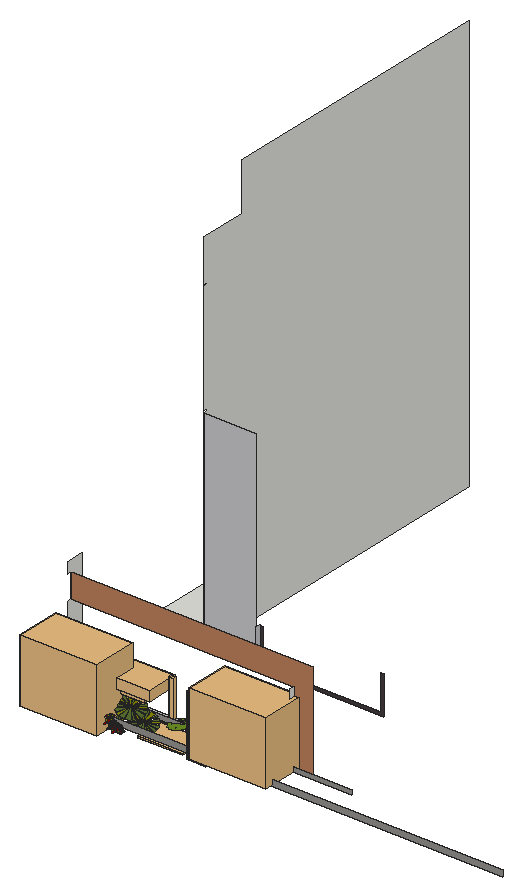
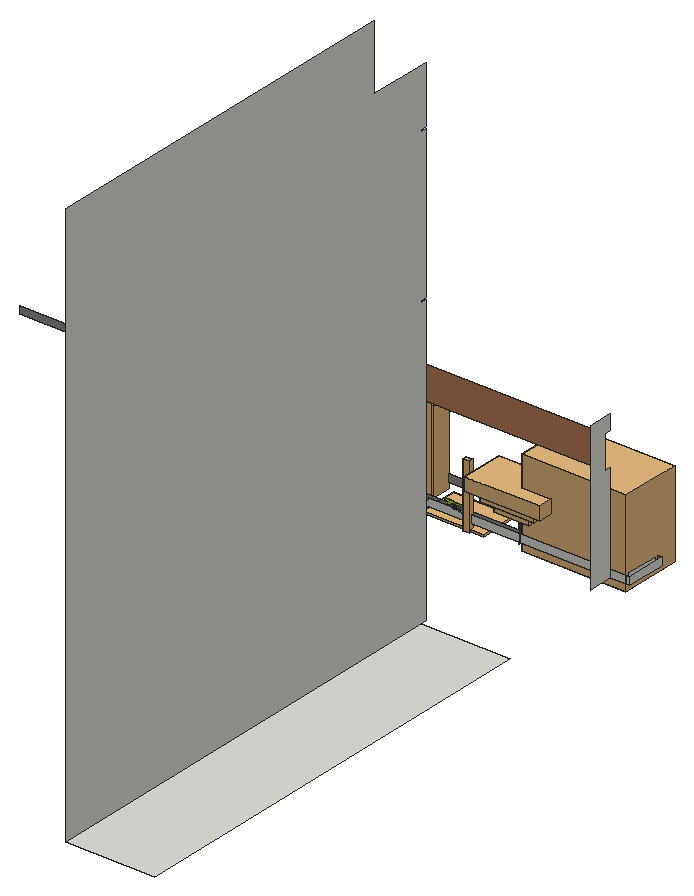
# SketchUp Ruby script. Lengths in inches.
U = 1.inch
M = Sketchup.active_model
def pt(a) = Geom::Point3d.new(a.map { |v| v * U })
def face(e, loops, mat)
  f = e.add_face(loops[0].map { |a| pt(a) })
  loops[1..].each { |l| e.add_face(l.map { |a| pt(a) }).erase! }
  f.material = f.back_material = mat if mat
  f
end
# faces: each face lists its corners as indices into pts; further lists are holes
def faces(e, pts, list, mat = nil) = list.each { |f| face(e, (f[0].is_a?(Array) ? f : [f]).map { |l| l.map { |i| pts[i] } }, mat) }
# xy, xz, yz: faces in a plane at the given z, y or x. An outline is a flat list of corners, or four numbers for a rectangle; further outlines are holes
def ring(l) = l.size == 4 ? [[l[0], l[1]], [l[2], l[1]], [l[2], l[3]], [l[0], l[3]]] : l.each_slice(2).to_a
def flat(e, list, mat, &to3) = list.each { |f| face(e, (f[0].is_a?(Array) ? f : [f]).map { |l| ring(l).map { |u, v| to3.(u, v) } }, mat) }
def xy(e, z, list, mat = nil) = flat(e, list, mat) { |x, y| [x, y, z] }
def xz(e, y, list, mat = nil) = flat(e, list, mat) { |x, z| [x, y, z] }
def yz(e, x, list, mat = nil) = flat(e, list, mat) { |y, z| [x, y, z] }
def lines(e, pts, list) = list.each { |a, b| e.add_line(pt(pts[a]), pt(pts[b])) }
# prism: a flat outline (further loops are holes) pulled along v
def prism(e, loops, v, mat = nil)
  f = face(e, loops, mat); d = Geom::Vector3d.new(v.map { |x| x * U })
  f.pushpull(f.normal.samedirection?(d) ? d.length : -d.length)
end
def box(e, o, s, mat = nil) = prism(e, [[o, [o[0] + s[0], o[1], o[2]], [o[0] + s[0], o[1] + s[1], o[2]], [o[0], o[1] + s[1], o[2]]]], [0, 0, s[2]], mat)
def at(x, y, z, deg = 0) = Geom::Transformation.translation(pt([x, y, z])) * Geom::Transformation.rotation(ORIGIN, Z_AXIS, deg.degrees)
def axes(o, x, y, z) = Geom::Transformation.new([*x, 0, *y, 0, *z, 0, *pt(o).to_a, 1])
def part(name) = M.definitions.add(name)
# library, detail: a bought-in or finely detailed component or shape, given as its bounding box
def library(name, o, s) = part(name).tap { |d| box(d.entities, o, s) }
def detail(e, o, s) = box(e.add_group.entities, o, s)
def put(e, d, t, mat = nil) = e.add_instance(d, t).tap { |i| i.material = mat if mat }
def group(e, t, mat = nil) = e.add_group.tap { |g| g.transformation = t; g.material = mat if mat }.entities
root = M.entities
M.materials.add("[0022_Maroon]").color = [128, 0, 0]
M.materials.add("[0043_SaddleBrown]").color = [139, 69, 19]
M.materials.add("[0058_Olive]").color = [128, 128, 0]
M.materials.add("[0059_DarkOliveGreen]").color = [85, 107, 47]
M.materials.add("[0061_OliveDrab]").color = [107, 142, 35]
M.materials.add("[Asphalt New]").color = [67, 60, 62]
M.materials.add("[Granite Light Gray]").color = [149, 148, 144]
M.materials.add("[Polished Concrete New]").color = [200, 200, 203]
M.materials.add("[Wood Veneer 02]").color = [190, 128, 91]
c1 = library("EXOTIC-KENTIA\#1",[0.7,-0.7,-0.11],[104.19,106.14,86.09])
c2 = part("Group\#46")
p = [[0.46,5.4,1.48],[0.55,4.86,1.35],[0.68,4.33,1.23],[0.85,3.8,1.12],[1.04,3.28,1.02],[1.28,2.78,0.93],
  [1.54,2.29,0.84],[1.84,1.82,0.77],[2.17,1.36,0.71],[2.52,0.93,0.66],[2.91,0.52,0.62],[2.91,0,0.48],
  [2.47,0.44,0.52],[2.06,0.9,0.56],[1.68,1.39,0.625],[1.34,1.9,0.7],[1.03,2.43,0.79],[0.76,2.98,0.89],
  [0.53,3.55,1],[0.34,4.13,1.12],[0.19,4.72,1.25],[0.09,5.3125,1.39],[0.02,5.91,1.54],[0,6.51,1.69],
  [0.02,6.88,1.8],[0.1,7.24,1.91],[0.22,7.59,2.02],[0.39,7.92,2.14],[0.6,8.22,2.26],[0.85,8.49,2.38],
  [1.14,8.72,2.49],[1.45,8.91,2.6],[1.8,9.0625,2.71],[2.16,9.17,2.8],[2.53,9.22,2.88],[2.91,9.23,2.95],
  [2.91,4.61,1.72],[2.68,3.89,1.48],[2.18,2.26,0.95],[2.59,5.625,1.93],[1.61,4.02,1.32],[2.34,6.73,2.18],
  [1.25,5.66,1.69],[2.4,7.87,2.5],[1.14,7.72,2.22],[2.4375,8.83,2.76],[2.16,8.77,2.69],[1.89,8.68,2.62],
  [1.625,8.56,2.54],[1.39,8.42,2.46],[1.16,8.24,2.37],[0.97,8.04,2.28],[0.79,7.82,2.19],[0.65,7.58,2.1],
  [0.54,7.32,2.01],[0.45,7.05,1.92],[0.4,6.78,1.84],[0.39,6.49,1.76],[0.41,5.95,1.62],[5.79,6.88,1.8],
  [5.82,6.51,1.69],[5.79,5.91,1.54],[5.73,5.3125,1.39],[5.625,4.72,1.25],[5.48,4.13,1.12],[5.29,3.55,1],
  [5.06,2.98,0.89],[4.79,2.43,0.79],[4.48,1.9,0.7],[4.14,1.39,0.625],[3.76,0.9,0.56],[3.35,0.44,0.52],
  [3.29,0.93,0.66],[3.65,1.36,0.71],[3.98,1.82,0.77],[4.27,2.29,0.84],[4.54,2.78,0.93],[4.77,3.28,1.02],
  [4.97,3.8,1.12],[5.13,4.33,1.23],[5.26,4.86,1.35],[5.35,5.4,1.48],[5.41,5.95,1.62],[5.43,6.49,1.76],
  [5.41,6.78,1.84],[5.36,7.05,1.92],[5.28,7.32,2.01],[5.16,7.58,2.1],[5.02,7.82,2.19],[4.85,8.04,2.28],
  [4.65,8.24,2.37],[4.43,8.42,2.46],[4.1875,8.56,2.54],[3.93,8.68,2.62],[3.66,8.77,2.69],[3.38,8.83,2.76],
  [4.67,7.72,2.22],[3.41,7.87,2.5],[4.5625,5.66,1.69],[3.47,6.73,2.18],[4.21,4.02,1.32],[3.23,5.625,1.93],
  [3.64,2.26,0.95],[3.13,3.89,1.48],[3.29,9.22,2.88],[3.66,9.17,2.8],[4.02,9.0625,2.71],[4.36,8.91,2.6],
  [4.68,8.72,2.49],[4.96,8.49,2.38],[5.21,8.22,2.26],[5.43,7.92,2.14],[5.59,7.59,2.02],[5.72,7.24,1.91],
  [2.91,14.34,0]]
faces(c2.entities,p,[[0,1,2,3,4,5,6,7,8,9,10,11,12,13,14,15,16,17,18,19,20,21,22,23,24,25,26,27,28,29,30,31,32,33,34,35,36,10,37,38,39,40,41,42,43,44,45,46,47,48,49,50,51,52,53,54,55,56,57,58],[59,60,61,62,63,64,65,66,67,68,69,70,71,11,10,72,73,74,75,76,77,78,79,80,81,82,83,84,85,86,87,88,89,90,91,92,93,94,95,96,97,98,99,100,101,102,103,10,36,35,104,105,106,107,108,109,110,111,112,113]],"[0022_Maroon]")
faces(c2.entities,p,[[43,42,41,40,39,38,37,10,9,8,7,6,5,4,3,2,1,0,58,57,56,55,54,53,52,51,50,49,48,47,46,45,44],[99,98,97,96,95,94,93,92,91,90,89,88,87,86,85,84,83,82,81,80,79,78,77,76,75,74,73,72,10,103,102,101,100]],"[0058_Olive]")
lines(c2.entities,p,[[35,114]])
c3 = part("EXOTIC-CROTON")
p = [[0,0,13.11],[0,0,0],[0,0,17.6]]
lines(c3.entities,p,[[0,1],[0,2]])
put(c3.entities,c2,at(-2.91,-14.34,9.43),"[0058_Olive]")
put(c3.entities,c2,at(-13.875,-4.65,9.43,-60),"[0058_Olive]")
put(c3.entities,c2,at(-10.97,9.69,9.43,-120),"[0058_Olive]")
put(c3.entities,c2,at(2.91,14.34,9.43,180),"[0058_Olive]")
put(c3.entities,c2,at(13.875,4.65,9.43,120),"[0058_Olive]")
put(c3.entities,c2,at(10.97,-9.69,9.43,60),"[0058_Olive]")
put(c3.entities,c2,axes([-3.96,11.79,13.11],[-0.73612,-0.425,0],[0.425,-0.73612,0],[0,0,0.85]),"[0058_Olive]")
put(c3.entities,c2,axes([8.24,9.32,13.11],[-0.73612,0.425,0],[-0.425,-0.73612,0],[0,0,0.85]),"[0058_Olive]")
put(c3.entities,c2,axes([3.96,-11.79,13.11],[0.73612,0.425,0],[-0.425,0.73612,0],[0,0,0.85]),"[0058_Olive]")
put(c3.entities,c2,axes([-8.24,-9.32,13.11],[0.73612,-0.425,0],[0.425,0.73612,0],[0,0,0.85]),"[0058_Olive]")
put(c3.entities,c2,axes([12.19,-2.47,13.11],[0,0.85,0],[-0.85,0,0],[0,0,0.85]),"[0058_Olive]")
put(c3.entities,c2,axes([-12.19,2.47,13.11],[0,-0.85,0],[0.85,0,0],[0,0,0.85]),"[0058_Olive]")
put(c3.entities,c2,axes([1.98,9.75,17.6],[-0.68,0,0],[0,-0.68,0],[0,0,0.68]),"[0058_Olive]")
put(c3.entities,c2,axes([7.46,-6.59,17.6],[0.34,0.5889,0],[-0.5889,0.34,0],[0,0,0.68]),"[0058_Olive]")
put(c3.entities,c2,axes([9.4375,3.16,17.6],[-0.34,0.5889,0],[-0.5889,-0.34,0],[0,0,0.68]),"[0058_Olive]")
put(c3.entities,c2,axes([-9.4375,-3.16,17.6],[0.34,-0.5889,0],[0.5889,0.34,0],[0,0,0.68]),"[0058_Olive]")
put(c3.entities,c2,axes([-7.46,6.59,17.6],[-0.34,-0.5889,0],[0.5889,-0.34,0],[0,0,0.68]),"[0058_Olive]")
put(c3.entities,c2,axes([-1.98,-9.75,17.6],[0.68,0,0],[0,0.68,0],[0,0,0.68]),"[0058_Olive]")
c4 = part("Group\#44")
p = [[12.14,1.93,0.52],[12.15,1.96,0.53]]
lines(c4.entities,p,[[0,1]])
detail(c4.entities,[0,0,0],[22.29,22.29,3.9])
c5 = part("EXOTIC-BUSHY-02")
prism(c5.entities,[[[-0.2,0.11,-0.03],[-0.16,0.16,-0.03],[-0.11,0.2,-0.03],[-0.06,0.22,-0.03],[0,0.23,-0.03],[0.06,0.22,-0.03],[0.11,0.2,-0.03],[0.16,0.16,-0.03],[0.2,0.11,-0.03],[0.22,0.06,-0.03],[0.23,0,-0.03],[0.22,-0.06,-0.03],[0.2,-0.11,-0.03],[0.16,-0.16,-0.03],[0.11,-0.2,-0.03],[0.06,-0.22,-0.03],[0,-0.23,-0.03],[-0.06,-0.22,-0.03],[-0.11,-0.2,-0.03],[-0.16,-0.16,-0.03],[-0.2,-0.11,-0.03],[-0.22,-0.06,-0.03],[-0.23,0,-0.03],[-0.22,0.06,-0.03]]],[0,0,12.79],"[0043_SaddleBrown]")
put(c5.entities,c4,axes([-11.15,-11.15,16.66],[1,0,0],[0,1,0],[0,0,-1]))
put(c5.entities,c4,axes([-7.91,-7.91,13.14],[0.71,0,0],[0,0.71,0],[0,0,-0.71]))
put(c5.entities,c4,axes([-5.11,-5.11,9.7],[0.4588,0,0],[0,0.4588,0],[0,0,-0.4588]))
c6 = part("Group\#77")
p = [[9.84,8.91,4.16],[6.8,0.43,0.2],[7.02,0.37,0.17],[7.24,0.3125,0.15],[7.46,0.26,0.12],[7.68,0.21,0.1],
  [7.91,0.17,0.08],[8.13,0.13,0.0625],[8.36,0.1,0.04],[8.59,0.07,0.03],[8.8125,0.04,0.02],[9.04,0.02,0.01],
  [9.27,0.01,0],[9.5,0,0],[10.87,0.04,0.02],[11.1,0.07,0.03],[11.33,0.1,0.04],[11.55,0.13,0.0625],
  [11.78,0.17,0.08],[12,0.21,0.1],[12.22,0.26,0.12],[12.45,0.3125,0.15],[12.67,0.37,0.17],[12.88,0.43,0.2],
  [13.1,0.5,0.23],[13.32,0.57,0.27],[13.53,0.64,0.3],[4.34,1.52,0.71],[4.43,1.46,0.68],[4.53,1.41,0.66],
  [4.625,1.35,0.63],[4.72,1.3,0.6],[4.82,1.24,0.58],[4.92,1.19,0.55],[5.02,1.14,0.53],[5.12,1.09,0.51],
  [5.22,1.04,0.48],[5.32,0.99,0.46],[5.43,0.94,0.44],[5.53,0.9,0.42],[14.76,1.19,0.55],[14.86,1.24,0.58],
  [14.96,1.3,0.6],[15.06,1.35,0.63],[15.16,1.41,0.66],[15.25,1.46,0.68],[15.35,1.52,0.71],[15.44,1.58,0.74],
  [15.53,1.64,0.76],[15.63,1.7,0.79],[15.72,1.76,0.82],[15.8125,1.82,0.85],[15.9,1.89,0.88],[1.5,4.1875,1.95],
  [1.62,4.01,1.87],[1.75,3.84,1.79],[1.88,3.67,1.71],[2.02,3.51,1.63],[2.16,3.34,1.56],[2.3,3.18,1.48],
  [2.45,3.02,1.41],[2.61,2.87,1.34],[2.76,2.72,1.27],[2.92,2.57,1.2],[3.09,2.43,1.13],[3.26,2.29,1.07],
  [17.81,3.67,1.71],[17.74,3.59,1.67],[17.67,3.51,1.63],[17.6,3.42,1.6],[17.53,3.34,1.56],[17.46,3.26,1.52],
  [17.38,3.18,1.48],[17.31,3.1,1.45],[17.23,3.02,1.41],[17.16,2.95,1.375],[17.08,2.87,1.34],[17,2.79,1.3],
  [16.92,2.72,1.27],[18.53,4.73,2.2],[18.64,4.91,2.29],[18.74,5.1,2.38],[18.83,5.29,2.47],[18.92,5.48,2.55],
  [19.01,5.67,2.64],[19.09,5.86,2.73],[19.17,6.06,2.83],[19.24,6.26,2.92],[19.3,6.46,3.01],[19.36,6.66,3.1],
  [19.42,6.86,3.2],[19.47,7.06,3.29],[0.1,7.67,3.58],[0.13,7.47,3.48],[0.17,7.26,3.39],[0.22,7.06,3.29],
  [0.27,6.86,3.2],[0.32,6.66,3.1],[0.38,6.46,3.01],[0.45,6.26,2.92],[0.52,6.06,2.83],[0.59,5.86,2.73],
  [0.67,5.67,2.64],[0.76,5.48,2.55],[0.85,5.29,2.47],[19.66,8.29,3.87],[19.67,8.5,3.96],[19.68,8.71,4.06],
  [19.69,8.91,4.16],[19.68,9.12,4.25],[19.67,9.33,4.35],[19.66,9.54,4.45],[19.64,9.74,4.54],[19.62,9.95,4.64],
  [19.59,10.16,4.74],[19.55,10.36,4.83],[19.51,10.57,4.93],[19.47,10.77,5.02],[0.1,10.16,4.74],[0.08,10.05,4.6875],
  [0.07,9.95,4.64],[0.05,9.85,4.59],[0.04,9.74,4.54],[0.03,9.64,4.5],[0.02,9.54,4.45],[0.02,9.43,4.4],
  [0.01,9.33,4.35],[0.01,9.23,4.3],[0,9.12,4.25],[0,9.02,4.21],[0,8.91,4.16],[0.85,12.54,5.85],
  [0.8,12.45,5.8],[0.76,12.35,5.76],[0.72,12.26,5.72],[0.67,12.16,5.67],[0.63,12.0625,5.625],[0.59,11.97,5.58],
  [0.56,11.87,5.53],[0.52,11.77,5.49],[0.48,11.67,5.44],[0.45,11.57,5.4],[0.41,11.47,5.35],[0.38,11.375,5.3],
  [3.26,15.54,7.25],[3.09,15.4,7.18],[2.92,15.26,7.12],[2.76,15.11,7.05],[2.61,14.96,6.98],[2.45,14.81,6.9],
  [2.3,14.65,6.83],[2.16,14.49,6.76],[2.02,14.32,6.68],[1.88,14.16,6.6],[1.75,13.99,6.52],[1.62,13.82,6.44],
  [1.5,13.64,6.36],[6.8,17.4,8.11],[6.58,17.33,8.08],[6.37,17.26,8.05],[6.16,17.1875,8.01],[5.94,17.11,7.98],
  [5.73,17.02,7.9375],[5.53,16.93,7.9],[5.32,16.84,7.85],[5.12,16.74,7.81],[4.92,16.64,7.76],[4.72,16.53,7.71],
  [4.53,16.42,7.66],[4.34,16.31,7.61],[9.5,17.83,8.3125],[9.38,17.83,8.3125],[9.27,17.82,8.31],[9.16,17.8125,8.31],
  [9.04,17.81,8.3],[8.93,17.8,8.3],[8.8125,17.79,8.29],[8.7,17.77,8.29],[8.59,17.76,8.28],[8.47,17.75,8.28],
  [8.36,17.73,8.27],[8.25,17.72,8.26],[8.13,17.7,8.25],[19.09,11.97,5.58],[19.05,12.0625,5.625],[19.01,12.16,5.67],
  [18.97,12.26,5.72],[18.92,12.35,5.76],[18.88,12.45,5.8],[18.83,12.54,5.85],[18.79,12.64,5.89],[18.74,12.73,5.9375],
  [18.6875,12.83,5.98],[18.64,12.92,6.02],[18.59,13.01,6.07],[18.53,13.1,6.11],[16.92,15.11,7.05],[17,15.04,7.01],
  [17.08,14.96,6.98],[17.16,14.88,6.94],[17.23,14.81,6.9],[17.31,14.73,6.87],[17.38,14.65,6.83],[17.46,14.57,6.79],
  [17.53,14.49,6.76],[17.6,14.41,6.72],[17.67,14.32,6.68],[17.74,14.24,6.64],[17.81,14.16,6.6],[15.9,15.94,7.43],
  [15.8125,16.01,7.46],[15.72,16.07,7.49],[15.63,16.13,7.52],[15.53,16.19,7.55],[15.44,16.25,7.58],[15.35,16.31,7.61],
  [15.25,16.37,7.63],[15.16,16.42,7.66],[15.06,16.48,7.68],[14.96,16.53,7.71],[14.86,16.59,7.73],[14.76,16.64,7.76],
  [13.53,17.1875,8.01],[13.32,17.26,8.05],[13.1,17.33,8.08],[12.88,17.4,8.11],[12.67,17.46,8.14],[12.45,17.52,8.17],
  [12.22,17.57,8.19],[12,17.62,8.22],[11.78,17.66,8.24],[11.55,17.7,8.25],[11.33,17.73,8.27],[11.1,17.76,8.28],
  [10.87,17.79,8.29]]
faces(c6.entities,p,[[0,1,2,3,4,5,6,7,8,9,10,11,12,13],[0,14,15,16,17,18,19,20,21,22,23,24,25,26],[0,40,41,42,43,44,45,46,47,48,49,50,51,52],[0,53,54,55,56,57,58,59,60,61,62,63,64,65],[0,79,80,81,82,83,84,85,86,87,88,89,90,91],[0,92,93,94,95,96,97,98,99,100,101,102,103,104],[0,105,106,107,108,109,110,111,112,113,114,115,116,117],[0,118,119,120,121,122,123,124,125,126,127,128,129,130],
  [0,144,145,146,147,148,149,150,151,152,153,154,155,156],[0,170,171,172,173,174,175,176,177,178,179,180,181,182],[0,196,197,198,199,200,201,202,203,204,205,206,207,208],[0,209,210,211,212,213,214,215,216,217,218,219,220,221]],"[0059_DarkOliveGreen]")
faces(c6.entities,p,[[0,27,28,29,30,31,32,33,34,35,36,37,38,39],[0,66,67,68,69,70,71,72,73,74,75,76,77,78],[0,131,132,133,134,135,136,137,138,139,140,141,142,143],[0,157,158,159,160,161,162,163,164,165,166,167,168,169],[0,183,184,185,186,187,188,189,190,191,192,193,194,195],[0,222,223,224,225,226,227,228,229,230,231,232,233,234]],"[0058_Olive]")
c7 = part("EXOTIC-AUS-PALM")
put(c7.entities,c6,axes([-13.78,-12.48,-5.82],[1.4,0,0],[0,1.4,0],[0,0,1.4]))
put(c7.entities,c6,at(-21.65,-8.91,-12.03))
put(c7.entities,c6,axes([-1.28,-11.86,-13.4],[1.33,0,0],[0,1.33,0],[0,0,1.33]))
c8 = library("EXOTIC-BULLRUSH",[-0.59,-0.59,-0.94],[7.09,7.09,64.29])
c9 = library("EXOTIC-AMAZON-LILY",[-1.1,-0.12,0],[60.56,66.69,1.97])
c10 = library("EXOTICA-CAT-TAIL",[-18.64,-20.64,0],[26.41,31.25,82.25])
c11 = library("EXOTIC-BAMBOO-TOO",[-9.25,-15.15,0],[30.31,37.46,85.46])
c12 = library("EXOTIC-BAMBOO",[-8.14,-8.14,0],[38.48,34.74,73.65])
c13 = library("EXOTIC-PEONY",[-0.63,-0.48,-0.08],[13.23,10.24,55.71])
c14 = library("EXOTIC-RED-POKER\#1",[-1.18,-1.18,0],[10.24,10.24,66.04])
xy(root,0,[[0,304.24,88.9375,747.375]])
xz(root,114.25,[[0,0,641.18,7.8125]],"[Granite Light Gray]")
xz(root,150.16,[[3.82,0.6875,408.3,7.8125]],"[Granite Light Gray]")
xz(root,153.99,[[0,0,20.0625,7.8125],[20.0625,0,321.78,7.8125]])
xz(root,160.36,[[321.78,0,347.76,0,347.76,131.1875,20.0625,131.1875,20.0625,97.93,321.78,97.93]],"[Wood Veneer 02]")
xz(root,298.43,[[88.9375,0,160.07,287.46]],"[Polished Concrete New]")
xz(root,304.24,[[160.07,0,328.15,0,328.15,52.25,323.93,52.25,323.93,4.22,164.29,4.22,164.29,52.25,160.07,52.25]],"[Asphalt New]")
yz(root,0,[[114.25,0,153.99,7.8125]])
yz(root,3.82,[[118.08,0.6875,150.16,7.8125]])
yz(root,20.0625,[[153.99,0,153.99,97.93,160.36,97.93,160.36,131.1875,153.99,131.1875,153.99,146.4375,178.37,146.4375,178.37,0]])
yz(root,88.9375,[[298.43,0,298.43,287.46,304.24,287.46,304.24,289.58,298.43,289.58,298.43,440.86,304.24,440.86,304.24,442.55,298.43,442.55,298.43,500.25,363.07,500.25,363.07,566.3125,747.375,566.3125,747.375,0]])
yz(root,160.07,[[298.43,0,304.24,52.25]],"[Polished Concrete New]")
yz(root,321.78,[[153.99,0,160.36,97.93]])
p = [[193.92,154,8.05],[192.73,153.86,8.3],[192.01,151.875,7.59],[192.05,150.6875,7.05],[192.66,150,6.58],[193.37,149.66,6.25],
  [192.67,148.58,5.94],[193.09,147.58,5.39],[193.85,147.02,4.9375],[195.28,146.53,4.35],[195.76,146.3,4.125],[195.85,147.5,4.64],
  [196.51,148.72,5.02],[197.52,149.89,5.28],[198.78,150.74,5.34],[199.17,150.9,5.3125],[199.31,150.84,5.25],[199.15,150.55,5.16],
  [197.87,149.16,4.87],[197.03,147.93,4.53],[196.34,146.61,4.12],[196.13,145.91,3.85],[196.44,145.3,3.5],[197.15,144.97,3.17],
  [198.34,144.62,2.71],[199.42,144.32,2.29],[199.98,144.17,2.08],[200.91,143.625,1.6],[201.99,143.24,1.15],[203.08,143.01,0.76],
  [203.66,142.85,0.54],[203.58,143.52,0.86],[203.47,144.52,1.34],[204.58,142.73,0.25],[204.89,142.51,0.08],[205.9,142.45,-0.21],
  [206.92,142.39,-0.5],[209.25,142.85,-0.89],[212.55,143.08,-1.64],[213.89,144.1875,-1.49],[215.22,144.97,-1.48],[216.08,145.4,-1.51],
  [214.42,146.54,-0.57],[213.12,147.16,0.04],[211.25,147.59,0.72],[209.94,147.85,1.17],[209.29,148.16,1.48],[208.77,148.41,1.72],
  [208.77,148.58,1.8],[209.125,148.63,1.73],[210.16,148.5,1.41],[211.04,148.28,1.08],[212.85,147.59,0.31],[214.37,146.96,-0.37],
  [215.33,146.62,-0.77],[215.96,146.21,-1.11],[216.43,145.78,-1.43],[217.11,146.45,-1.3],[217.43,147.02,-1.13],[217.6,147.54,-0.94],
  [217.68,147.94,-0.78],[217.85,148.42,-0.61],[216.36,149.31,0.17],[214.95,149.78,0.75],[213.71,150,1.16],[211.41,150.24,1.87],
  [209.65,150.3125,2.35],[208.16,150.42,2.78],[207.05,150.5625,3.13],[206.52,150.81,3.38],[206.49,151.15,3.54],[207.32,151.3,3.39],
  [208.46,151.39,3.14],[210.46,151.22,2.55],[212.61,150.79,1.8],[214.99,150.12,0.89],[217.67,149.09,-0.26],[217.97,150.81,0.43],
  [218.01,151.83,0.88],[217.59,152.27,1.1875],[216.61,152.74,1.65],[215.4,153.01,2.08],[213.78,153.12,2.55],[212.4,153.19,2.93],
  [210.36,153.28,3.5],[208.85,153.22,3.86],[207.67,153.17,4.14],[207.1,153.11,4.26],[206.77,153.26,4.42],[207.12,153.5,4.43],
  [207.99,153.81,4.34],[209.36,153.95,4.06],[212.13,153.83,3.29],[213.76,153.64,2.78],[215.21,153.38,2.3],[215.88,153.14,2.01],
  [217.22,152.74,1.49],[217.27,153.03,1.61],[216.9375,154.02,2.14],[216.59,154.9,2.625],[215.24,155.9,3.42],[213.83,156.09,3.87],
  [211.57,155.95,4.39],[209.58,155.53,4.71],[207.77,155.23,5.04],[206.97,155.07,5.18],[206.52,155.1,5.3],[206.57,155.28,5.37],
  [207.49,155.65,5.3],[209.72,156.18,4.96],[211.52,156.33,4.57],[214.4,156.32,3.83],[212.95,157.51,4.73],[211.49,158.13,5.39],
  [210.26,158.24,5.75],[209.625,158.04,5.82],[207.72,157.38,6.02],[206.31,156.77,6.11],[205.2,156.39,6.22],[204.75,156.35,6.32],
  [204.61,156.51,6.43],[204.85,156.68,6.44],[206.63,157.48,6.34],[208.06,157.93,6.18],[209.33,158.23,5.98],[210.3,158.43,5.83],
  [209.11,158.87,6.33],[208,159,6.67],[206.57,158.8125,6.96],[205.23,158.43,7.13],[203.86,158.16,7.36],[203.15,157.68,7.33],
  [201.97,157.09,7.37],[200.96,156.41,7.32],[200.48,155.5,7.04],[200.62,154.56,6.58],[200.96,154.01,6.25],[200.28,153.81,6.33],
  [199.7,154.26,6.68],[198.73,154.72,7.14],[197.46,154.69,7.45],[195.61,154.35,7.77],[197.42,152.83,6.63],[193.95,152.56,7.4],
  [196.18,152.94,7],[200.84,153.75,6.16],[201.41,154.45,6.33],[202.3125,155.95,6.77],[203.5,156.88,6.88],[204.52,157.43,6.86],
  [202.93,155.86,6.57],[202,154.56,6.22],[201.71,153.83,5.97],[203.01,154.99,6.16],[205.59,156.09,5.99],[207.64,156.66,5.72],
  [209.76,157.11,5.375],[210.83,157.25,5.16],[207.55,156.34,5.6],[205.6,155.7,5.8125],[203.45,154.83,5.97],[202.34,154.08,5.92],
  [201.88,153.66,5.85],[201.99,153.39,5.7],[202.34,153.34,5.59],[203.29,153.59,5.46],[204.25,154,5.39],[205.375,154.27,5.23],
  [208.64,154.79,4.62],[210.73,154.95,4.16],[212.68,154.8,3.59],[214.27,154.7,3.13],[214.86,154.42,2.85],[211.81,154.625,3.73],
  [210.08,154.56,4.15],[207.35,154.27,4.72],[204.94,153.77,5.11],[202.31,153.1,5.49],[203.68,152.03,4.66],[205.72,152.29,4.25],
  [207.64,152.49,3.85],[211.61,152.29,2.73],[213.58,151.92,2.06],[214.9,151.59,1.57],[215.52,151.3,1.28],[213.65,151.65,1.92],
  [210.58,151.96,2.85],[206.65,152.0625,3.91],[204.3,151.74,4.37],[206.4,149.69,2.91],[207.98,149.84,2.57],[209.92,149.64,1.98],
  [211.78,149.18,1.3],[213.18,148.7,0.72],[214.72,147.97,-0.01],[211.53,149,1.28],[209.69,149.42,1.94],[207.98,149.56,2.44],
  [206.42,149.45,2.8],[207.76,147.86,1.74],[209.47,147.57,1.17],[210.99,147.08,0.55],[212.24,146.48,-0.03],[212.79,145.9,-0.4375],
  [210.7,146.9,0.55],[209.13,147.3,1.13],[207.87,147.53,1.56],[209.17,146.29,0.67],[209.84,145.63,0.2],[210.82,144.78,-0.43],
  [210.64,144.89,-0.34],[208.76,146.14,0.7],[207.27,147.4,1.66],[206.14,148.92,2.63],[205.37,145.34,1.22],[205.38,149.42,3.05],
  [204.04,150.63,3.9375],[202.82,148.88,3.46],[201.58,146.05,2.51],[202.03,148.13,3.33],[202.94,150.0625,3.96],[203.68,151.08,4.23],
  [202.37,152.09,5.02],[200.23,149.89,4.58],[198.125,146.68,3.6875],[198.99,149.25,4.62],[200.47,150.95,5],[202.1,152.4,5.23],
  [201.66,152.82,5.53],[200.02,152.24,5.69],[197.84,151.48,5.91],[195.65,149.74,5.7],[197.15,151.3,6.01],[198.87,152.47,6.09],
  [200.81,152.92,5.8],[201.12,153.13,5.81],[200.48,153.43,6.11],[200.23,148.31,3.875],[200.96,149.49,4.22],[201.34,149.78,4.25],
  [201.61,149.85,4.21],[201.72,149.71,4.12],[201.5,149.24,3.97],[200.97,148.11,3.6],[200.4,146.87,3.1875],[199.96,145.5625,2.71],
  [199.73,144.95,2.5],[199.8,146.81,3.3125],[203.62,148.45,3.07],[203.97,148.875,3.17],[204.36,148.9,3.08],[204.58,148.71,2.9375],
  [204.61,148.3,2.74],[204.47,147.97,2.63],[203.96,146.66,2.17],[203.47,145.44,1.75],[203.4,147.3,2.61],[195.03,151.42,6.61],
  [196.01,151.94,6.59],[196.86,152.24,6.5],[197.32,152.21,6.375],[197.47,152.07,6.27],[196.04,151.18,6.24],[194.77,150.48,6.26],
  [194.4,150.35,6.29],[194.43,150.85,6.51],[204.02,153.2,5.09],[204.76,153.24,4.92],[205.3125,153.08,4.71],[205.26,152.86,4.625],
  [204.56,152.625,4.7],[203.7,152.68,4.94],[203.43,152.9375,5.13],[202.75,154.07,5.81],[203.51,154.26,5.7],[204.07,154.26,5.56],
  [204.05,154.04,5.46],[203.23,153.84,5.59],[202.625,153.82,5.73],[173.59,155.55,8.2],[171.69,155.95,7.89],[169.96,155.71,7.34],
  [168.98,155.28,6.89],[168.12,154.45,6.3],[167.73,154.18,6.08],[169.8125,154.125,6.59],[171.94,153.75,6.97],[173.99,153.17,7.23],
  [175.47,152.45,7.29],[175.75,152.22,7.26],[175.64,152.14,7.2],[175.13,152.23,7.11],[172.71,152.97,6.8125],[170.57,153.45,6.48],
  [168.27,153.85,6.07],[167.04,153.97,5.8],[165.99,153.79,5.45],[165.41,153.38,5.12],[164.79,152.7,4.66],[164.28,152.08,4.24],
  [164.02,151.76,4.03],[163.0625,151.22,3.55],[162.39,150.61,3.1],[161.98,149.98,2.71],[161.72,149.65,2.49],[162.875,149.7,2.8125],
  [164.63,149.76,3.29],[161.5,149.12,2.2],[161.125,148.94,2.03],[161.02,148.36,1.74],[160.91,147.78,1.45],[161.71,146.44,1.05],
  [162.11,144.55,0.3],[164.04,143.78,0.46],[165.4,143.02,0.47],[166.16,142.52,0.44],[168.14,143.48,1.38],[169.22,144.22,1.99],
  [169.97,145.29,2.66],[170.4375,146.05,3.12],[170.97,146.42,3.42],[171.4,146.72,3.67],[171.7,146.71,3.75],[171.79,146.51,3.68],
  [171.57,145.92,3.36],[171.18,145.42,3.03],[169.98,144.375,2.25],[168.88,143.51,1.58],[168.28,142.96,1.18],[167.57,142.59,0.83],
  [166.82,142.33,0.52],[167.99,141.93,0.65],[168.99,141.75,0.82],[169.88,141.65,1.01],[170.59,141.61,1.17],[171.43,141.51,1.34],
  [172.97,142.36,2.12],[173.79,143.17,2.7],[174.17,143.88,3.11],[174.6,145.21,3.82],[174.72,146.21,4.3],[174.91,147.07,4.73],
  [175.16,147.7,5.08],[175.6,148.01,5.33],[176.1875,148.02,5.49],[176.44,147.55,5.34],[176.6,146.89,5.09],[176.3,145.75,4.5],
  [175.56,144.51,3.75],[174.38,143.15,2.84],[172.58,141.61,1.68],[175.58,141.44,2.38],[177.36,141.42,2.83],[178.14,141.66,3.14],
  [178.96,142.22,3.6],[179.43,142.91,4.03],[179.61,143.84,4.49],[179.74,144.63,4.88],[179.9,145.8,5.45],[179.8,146.67,5.81],
  [179.71,147.35,6.09],[179.59,147.68,6.21],[179.87,147.87,6.37],[180.29,147.66,6.38],[180.8125,147.16,6.29],[181.07,146.375,6.01],
  [180.85,144.79,5.24],[180.52,143.86,4.73],[180.07,143.02,4.24],[179.65,142.64,3.96],[178.96,141.875,3.44],[179.46,141.84,3.56],
  [181.18,142.03,4.09],[182.72,142.23,4.57],[184.47,143.01,5.37],[184.8,143.82,5.82],[184.55,145.11,6.34],[183.82,146.25,6.66],
  [183.29,147.29,6.99],[183.02,147.75,7.125],[183.07,148.01,7.25],[183.38,147.98,7.32],[184.04,147.45,7.25],[184.95,146.17,6.91],
  [185.21,145.14,6.52],[185.2,143.49,5.77],[187.27,144.32,6.68],[188.36,145.16,7.34],[188.54,145.86,7.7],[188.19,146.23,7.77],
  [187.04,147.32,7.97],[185.99,148.13,8.06],[185.32,148.77,8.17],[185.24,149.02,8.27],[185.53,149.1,8.38],[185.82,148.96,8.39],
  [187.21,147.95,8.29],[188.01,147.125,8.13],[188.53,146.39,7.93],[188.88,145.84,7.78],[189.64,146.52,8.28],[189.87,147.16,8.62],
  [189.55,147.98,8.91],[188.87,148.75,9.08],[188.41,149.53,9.31],[187.57,149.94,9.28],[186.54,150.62,9.32],[185.35,151.2,9.27],
  [183.77,151.47,8.99],[182.13,151.39,8.53],[181.17,151.19,8.2],[180.82,151.59,8.28],[181.61,151.92,8.63],[182.42,152.48,9.09],
  [182.36,153.2,9.4],[181.76,154.26,9.72],[181.16,155.23,10],[180.9,155.92,10.24],[177.45,156.33,9.54],[175.38,156.31,9],
  [174.17,155.96,8.53],[168.39,152.82,5.63],[172.87,152.33,6.57],[175.84,151.48,6.95],[178.37,150.54,7.18],[179.1,150.79,7.48],
  [178.09,151.73,7.64],[176.76,152.98,7.86],[173.73,154.24,7.65],[176.45,153.38,7.96],[178.48,152.4,8.04],[179.27,151.28,7.74],
  [179.64,151.1,7.76],[180.16,151.47,8.06],[179.11,153.23,8.58],[178.64,155.22,9.35],[180.71,151.26,8.11],[181.93,150.9375,8.27],
  [184.54,150.42,8.71],[186.18,149.74,8.83],[187.125,149.15,8.8125],[184.39,150.07,8.52],[182.125,150.6,8.17],[180.86,150.77,7.92],
  [182.88,150.02,8.11],[184.79,148.54,7.9375],[185.8,147.36,7.67],[186.58,146.15,7.32],[186.82,145.54,7.11],[185.24,147.42,7.55],
  [184.12,148.54,7.76],[182.61,149.77,7.92],[181.29,150.41,7.87],[180.55,150.67,7.8],[180.09,150.61,7.65],[179.99,150.4,7.54],
  [180.44,149.86,7.41],[181.15,149.3125,7.34],[181.62,148.66,7.17],[182.53,146.79,6.57],[182.82,145.59,6.11],[182.55,144.47,5.53],
  [182.38,143.57,5.08],[181.88,143.22,4.8],[182.24,144.97,5.68],[182.13,145.96,6.09],[181.61,147.53,6.66],[180.76,148.91,7.0625],
  [179.58,150.42,7.4375],[177.72,149.64,6.61],[178.16,148.47,6.2],[178.53,147.37,5.8],[178.18,145.09,4.68],[177.52,143.96,4.01],
  [176.95,143.2,3.52],[176.44,142.85,3.23],[177.05,143.92,3.87],[177.6,145.68,4.8],[177.77,147.93,5.86],[177.21,149.28,6.32],
  [173.64,148.08,4.86],[173.91,147.17,4.52],[173.54,146.06,3.93],[172.76,144.99,3.24],[171.91,144.1875,2.67],[170.64,143.31,1.94],
  [172.4375,145.13,3.23],[173.17,146.1875,3.89],[173.41,147.17,4.39],[173.23,148.0625,4.74],[170.45,147.3,3.6875],[169.95,146.32,3.12],
  [169.08,145.44,2.5],[168.05,144.73,1.91],[167.04,144.41,1.51],[168.77,145.61,2.5],[169.46,146.51,3.08],[169.87,147.23,3.51],
  [167.71,146.49,2.62],[166.55,146.1,2.15],[165.08,145.54,1.52],[165.27,145.64,1.61],[167.44,146.72,2.65],[169.65,147.58,3.61],
  [172.29,148.23,4.58],[166.06,148.67,3.17],[173.16,148.66,5],[175.28,149.43,5.89],[172.22,150.13,5.41],[167.28,150.84,4.46],
  [170.92,150.58,5.28],[174.28,150.0625,5.91],[176.05,149.63,6.18],[177.82,150.39,6.97],[173.98,151.61,6.53],[171.23,151.61,5.82],
  [173.29,151.2,6.17],[173.8,150.98,6.2],[173.91,150.82,6.16],[173.68,150.76,6.07],[172.85,150.88,5.91],[170.89,151.1875,5.55],
  [168.72,151.52,5.14],[166.44,151.77,4.66],[165.37,151.9,4.44],[168.61,151.86,5.26],[171.48,149.67,5.02],[172.21,149.47,5.12],
  [172.26,149.25,5.03],[171.93,149.12,4.89],[171.21,149.1,4.69],[170.64,149.18,4.58],[168.35,149.48,4.125],[166.23,149.76,3.7],
  [169.48,149.8,4.56],[175.67,154.94,8.46],[176.65,154.59,8.56],[177.56,154.04,8.54],[178.08,153.54,8.45],[178.03,153.28,8.32],
  [177.79,153.2,8.22],[176.24,154.02,8.19],[175.02,154.75,8.2],[174.79,154.96,8.24],[179.17,148.73,6.57],[178.75,149.13,6.65],
  [178.85,149.62,6.89],[179.3,149.78,7.08],[179.75,149.44,7.04],[179.83,149.02,6.87],[179.56,148.7,6.66],[181.28,150.17,7.76],
  [181.6,149.74,7.65],[181.61,149.41,7.51],[181.22,149.42,7.41],[180.88,149.9,7.54],[180.85,150.24,7.68]]
faces(root,p,[[[0,1,2,3,4,5,6,7,8,9,10,11,12,13,14,15,16,17,18,19,20,21,22,23,24,25,26,27,28,29,30,31,32,33,34,35,36,37,38,39,40,41,42,43,44,45,46,47,48,49,50,51,52,53,54,55,56,57,58,59,60,61,62,63,64,65,66,67,68,69,70,71,72,73,74,75,76,77,78,79,80,81,82,83,84,85,86,87,88,89,90,91,92,93,94,95,80,96,97,98,99,100,101,102,103,104,105,106,107,108,109,110,111,112,113,114,115,116,117,118,119,120,121,122,123,124,125,126,127,128,129,130,131,132,133,134,135,136,137,138,139,140,141],[142,143,144,145,146,147,148,149,150,151,152,153,154,155,156,157,158,159,160,161,162,163,164,165,166,167,168,169,170,171,172,173,174,175,176,177,178,179,180,181,182,183,184,185,186,187,188,189,190,191,192,193,194,195,196,197,198,199,200,201,202,203,204,205,206,207,208,209,210,211,212,213,214,215,216,217,218,219,220,221,222,223,224,225,226,227,228,229,230,231,232,233,234,235,236],[237,238,239,240,241,242,243,244,245,246,247],[248,249,250,251,252,253,254,255,256],[257,258,259,260,261,262,263,264,265],[266,267,268,269,270,271,272],[273,274,275,276,277,278]],[[279,280,281,282,283,284,285,286,287,288,289,290,291,292,293,294,295,296,297,298,299,300,301,302,303,304,305,306,307,308,309,310,311,312,313,314,315,316,317,318,319,320,321,322,323,324,325,326,327,328,329,330,331,332,333,334,335,336,337,338,339,340,341,342,343,344,345,346,347,348,349,350,351,352,353,354,355,356,357,358,359,360,361,362,363,364,365,366,367,368,369,354,370,371,372,373,374,375,376,377,378,379,380,381,382,383,384,385,386,387,388,389,390,391,392,393,394,395,396,397,398,399,400,401,402,403,404,405,406,407,408,409,410,411,412,413,414,415,416,417,418,419,420],[421,422,423,424,425,426,427,428,429,430,431,432,433,434,435,436,437,438,439,440,441,442,443,444,445,446,447,448,449,450,451,452,453,454,455,456,457,458,459,460,461,462,463,464,465,466,467,468,469,470,471,472,473,474,475,476,477,478,479,480,481,482,483,484,485,486,487,488,489,490,491,492,493,494,495,496,497,498,499,500,501,502,503,504,505,506,507,508,509,510,511,512,513,514],[515,516,517,518,519,520,521,522,523,524,525],[526,527,528,529,530,531,532,533,534],[535,536,537,538,539,540,541,542,543],[544,545,546,547,548,549,550],[551,552,553,554,555,556]]],"[0061_OliveDrab]")
faces(root,p,[[143,142,236,235,234,233,232,231,230,229,228,227,226,225,224,223,222,221,220,219,218,217,216,215,214,213,212,211,210,209,208,207,206,205,204,203,202,201,200,199,198,197,196,195,194,193,192,191,190,189,188,187,186,185,184,183,182,181,180,179,178,177,176,175,174,173,172,171,170,169,168,167,166,165,164,163,162,161,160,159,158,157,156,155,154,153,152,151,150,149,148,147,146,145,144],[422,421,514,513,512,511,510,509,508,507,506,505,504,503,502,501,500,499,498,497,496,495,494,493,492,491,490,489,488,487,486,485,484,483,482,481,480,479,478,477,476,475,474,473,472,471,470,469,468,467,466,465,464,463,462,461,460,459,458,457,456,455,454,453,452,451,450,449,448,447,446,445,444,443,442,441,440,439,438,437,436,435,434,433,432,431,430,429,428,427,426,425,424,423]],"[0059_DarkOliveGreen]")
put(root,c1,axes([4,93.12,-7.125],[1,0,0],[0,0.5735,0],[0,0,1]))
put(root,c3,axes([94.78,108.43,-10.2],[0.783,0,0],[0,0.44905,0],[0,0,0.783]))
put(root,c3,axes([108.4,110.21,-7.125],[1,0,0],[0,0.5735,0],[0,0,1]))
put(root,c5,axes([116.76,146.41,-7.0625],[3.38,0,0],[0,1.93843,0],[0,0,3.38]))
put(root,c3,axes([122.3,108.43,-10.2],[0.783,0,0],[0,0.44905,0],[0,0,0.783]))
put(root,c7,axes([125.79,129,17.6875],[1.5,0,0],[0,0.86025,0],[0,0,1.5]))
put(root,c8,axes([159.23,152.41,-7.125],[1,0,0],[0,0.5735,0],[0,0,1]))
put(root,c9,axes([146.58,117.21,-7.125],[1,0,0],[0,0.5735,0],[0,0,1]))
put(root,c10,axes([232.93,124.64,-7.125],[1,0,0],[0,0.5735,0],[0,0,1]))
put(root,c11,axes([227.28,137.16,-7.125],[1,0,0],[0,0.5735,0],[0,0,1]))
put(root,c12,axes([242.99,129.34,-7.125],[1,0,0],[0,0.5735,0],[0,0,1]))
put(root,c13,axes([269.29,117.23,-7.125],[1,0,0],[0,0.5735,0],[0,0,1]))
put(root,c1,axes([223.93,104.12,0.6875],[1,0,0],[0,0.5735,0],[0,0,1]))
put(root,c14,axes([290.28,123.37,-7.125],[0,-0.5735,0],[1,0,0],[0,0,1]))
put(root,c3,axes([314.7,119.43,-2.38],[0.783,0,0],[0,0.44905,0],[0,0,0.783]))
